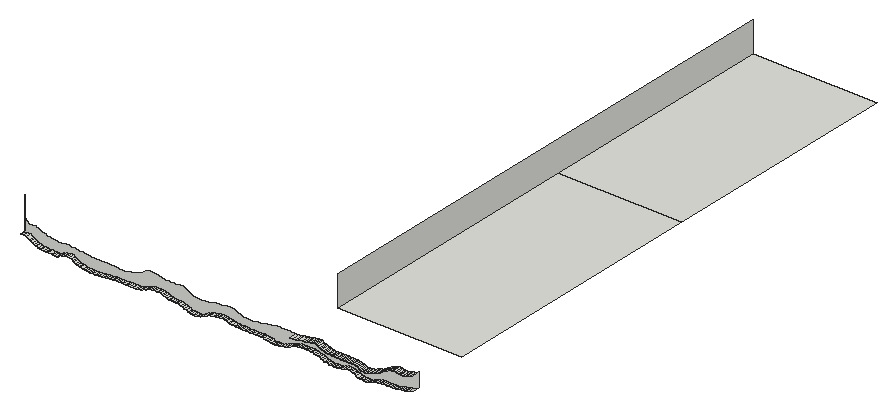
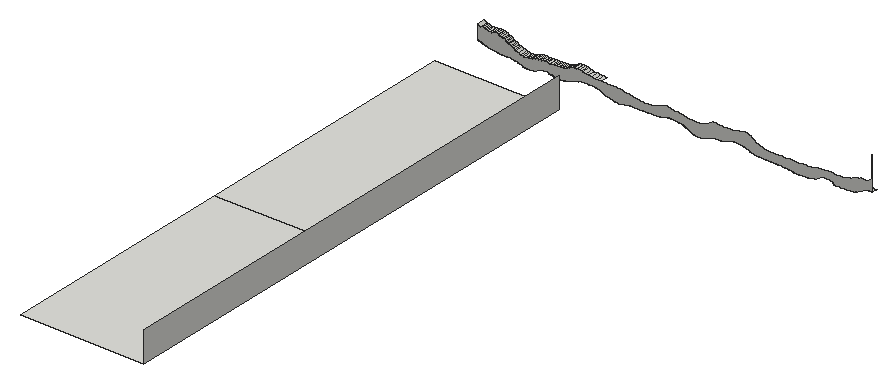
# SketchUp Ruby script. Lengths in inches.
U = 1.inch
M = Sketchup.active_model
def pt(a) = Geom::Point3d.new(a.map { |v| v * U })
def face(e, loops, mat)
  f = e.add_face(loops[0].map { |a| pt(a) })
  loops[1..].each { |l| e.add_face(l.map { |a| pt(a) }).erase! }
  f.material = f.back_material = mat if mat
  f
end
# faces: each face lists its corners as indices into pts; further lists are holes
def faces(e, pts, list, mat = nil) = list.each { |f| face(e, (f[0].is_a?(Array) ? f : [f]).map { |l| l.map { |i| pts[i] } }, mat) }
# xy, xz, yz: faces in a plane at the given z, y or x. An outline is a flat list of corners, or four numbers for a rectangle; further outlines are holes
def ring(l) = l.size == 4 ? [[l[0], l[1]], [l[2], l[1]], [l[2], l[3]], [l[0], l[3]]] : l.each_slice(2).to_a
def flat(e, list, mat, &to3) = list.each { |f| face(e, (f[0].is_a?(Array) ? f : [f]).map { |l| ring(l).map { |u, v| to3.(u, v) } }, mat) }
def xy(e, z, list, mat = nil) = flat(e, list, mat) { |x, y| [x, y, z] }
def xz(e, y, list, mat = nil) = flat(e, list, mat) { |x, z| [x, y, z] }
def yz(e, x, list, mat = nil) = flat(e, list, mat) { |y, z| [x, y, z] }
def lines(e, pts, list) = list.each { |a, b| e.add_line(pt(pts[a]), pt(pts[b])) }
# prism: a flat outline (further loops are holes) pulled along v
def prism(e, loops, v, mat = nil)
  f = face(e, loops, mat); d = Geom::Vector3d.new(v.map { |x| x * U })
  f.pushpull(f.normal.samedirection?(d) ? d.length : -d.length)
end
def box(e, o, s, mat = nil) = prism(e, [[o, [o[0] + s[0], o[1], o[2]], [o[0] + s[0], o[1] + s[1], o[2]], [o[0], o[1] + s[1], o[2]]]], [0, 0, s[2]], mat)
def at(x, y, z, deg = 0) = Geom::Transformation.translation(pt([x, y, z])) * Geom::Transformation.rotation(ORIGIN, Z_AXIS, deg.degrees)
def axes(o, x, y, z) = Geom::Transformation.new([*x, 0, *y, 0, *z, 0, *pt(o).to_a, 1])
def part(name) = M.definitions.add(name)
# library, detail: a bought-in or finely detailed component or shape, given as its bounding box
def library(name, o, s) = part(name).tap { |d| box(d.entities, o, s) }
def detail(e, o, s) = box(e.add_group.entities, o, s)
def put(e, d, t, mat = nil) = e.add_instance(d, t).tap { |i| i.material = mat if mat }
def group(e, t, mat = nil) = e.add_group.tap { |g| g.transformation = t; g.material = mat if mat }.entities
root = M.entities
xy(root,237.65,[[2918.33,2402.3,2919.02,2404.3],[2919.02,2402.3,2919.64,2404.3]])
xy(root,238.18,[[3012.28,2402.3,3012.96,2404.3]])
xy(root,238.33,[[2927.43,2402.3,2927.98,2404.3],[2927.98,2402.3,2928.66,2404.3]])
xy(root,238.34,[[2929.34,2402.3,2930.27,2404.3],[2930.27,2402.3,2930.76,2404.3],[2930.76,2402.3,2931.52,2404.3],[2931.52,2402.3,2932.15,2404.3],[2932.15,2402.3,2932.9,2404.3],
  [2932.9,2402.3,2933.52,2404.3],[2933.52,2402.3,2934.29,2404.3],[2934.29,2402.3,2934.91,2404.3]])
xy(root,238.62,[[2978.81,2402.3,2979.58,2404.3],[2979.58,2402.3,2980.21,2404.3],[2980.21,2402.3,2980.97,2404.3],[2980.97,2402.3,2981.59,2404.3],[2981.59,2402.3,2982.44,2404.3],
  [2982.44,2402.3,2983.08,2404.3],[2983.08,2402.3,2983.7,2404.3]])
xy(root,238.625,[[2977.39,2402.3,2978.25,2404.3]])
xy(root,238.89,[[3033.2,2402.3,3033.88,2404.3]])
xy(root,238.9,[[3034.64,2402.3,3035.26,2404.3],[3035.26,2402.3,3036.03,2404.3]])
xy(root,240.43,[[3001.48,2402.3,3002.05,2404.3]])
xy(root,241.52,[[2889.03,2402.3,2889.09,2404.3]])
xy(root,242.28,[[3019.3,2401.37,3019.8125,2404.3]])
xy(root,242.3,[[3017.54,2401.37,3018.21,2404.3]])
xy(root,242.33,[[3015.13,2401.37,3015.71,2404.3]])
xy(root,242.625,[[2994.64,2425.46,3043.1,2532.83],[2994.64,2532.83,3043.1,2628.15]])
xz(root,2404.3,[[2957.95,236.98,2957.34,237.01,2956.65,237.04,2955.89,237.11,2955.2,237.2,2954.67,237.33,2954,237.68,2953.0625,237.96,2952.5,238.28,2951.72,238.43,2950.94,238.78,2950.27,238.79,2949.73,238.8,2948.97,238.83,2948.22,238.875,2947.65,238.94,2947.07,239.04,2946.41,239.29,2945.83,239.53,2945.3,239.7,2944.61,239.92,2943.98,240.11,2943.2,240.27,2942.58,240.25,2941.875,240.23,2941.11,240.19,2940.4375,240.12,2939.78,240.03,2939.14,239.85,2938.59,239.52,2938.03,239.35,2937.44,239.18,2936.93,238.86,2936.24,238.72,2935.42,238.59,2934.91,238.34,2929.34,238.34,2928.66,238.33,2927.43,238.33,2926.71,238.32,2925.86,238.3,2925.23,238.28,2924.48,238.26,2923.85,238.15,2923.09,238.13,2922.54,238.1,2921.6875,237.98,2921.07,237.94,2920.31,237.89,2919.64,237.65,2918.33,237.65,2917.64,237.66,2916.89,237.67,2916.29,237.68,2915.68,237.71,2914.97,237.76,2914.28,237.82,2913.62,237.9,2912.68,238.21,2912.21,238.31,2911.3,238.43,2910.65,238.74,2910.07,239.11,2909.49,239.38,2909.03,239.71,2908.33,240.11,2907.64,240.09,2906.98,240.05,2906.39,239.99,2905.66,239.88,2905.11,239.69,2904.53,239.55,2903.97,238.9375,2903.44,238.77,2902.7,238.79,2901.83,238.8,2901.32,238.82,2900.28,238.92,2899.59,238.93,2898.89,238.94,2898.19,238.97,2897.51,239.03,2896.82,239.09,2896.04,239.19,2895.53,239.52,2894.97,239.64,2894.52,239.86,2893.73,240.2,2893.13,240.59,2892.59,240.85,2891.57,241.55,2890.3,241.69,2889.09,241.52,2889.09,246.2,2890.66,244.96,2892.05,244.9375,2893.3,244.92,2893.52,244.61,2894.08,244.54,2894.84,244.41,2895.51,244.11,2896.03,243.95,2896.69,243.79,2897.21,243.48,2897.85,243.3,2898.4375,243.14,2898.92,243.06,2899.64,242.85,2900.22,242.78,2901.03,242.73,2901.57,242.68,2902.24,242.51,2902.76,242.46,2903.3,242.58,2903.93,242.57,2904.56,242.81,2905.13,242.86,2905.69,242.89,2906.33,242.92,2906.76,242.625,2907.37,242.65,2907.92,242.62,2908.55,242.58,2909.11,242.57,2909.75,242.48,2910.41,242.38,2911.07,242.34,2911.74,242.24,2912.91,241.96,2913.68,241.89,2914.5,241.83,2915.1,241.78,2915.87,241.75,2916.32,241.74,2916.87,241.72,2918.13,241.7,2918.86,241.69,2919.53,241.68,2920.12,241.68,2920.61,241.67,2921.3125,241.74,2921.88,241.75,2923.88,241.75,2924.37,241.67,2924.9,241.66,2925.51,241.57,2926.05,241.53,2926.67,241.51,2927.22,241.49,2927.92,241.48,2928.58,241.47,2929.15,241.46,2929.86,241.6,2930.59,241.85,2931.26,241.91,2932.16,242.1,2932.93,242.46,2933.63,242.78,2934.4,242.97,2934.93,243.23,2935.33,243.48,2935.85,243.72,2936.1875,244.12,2936.66,244.39,2937.14,244.73,2937.625,244.87,2938.21,244.95,2938.89,245.01,2939.54,244.81,2940.11,244.7,2940.59,244.67,2941.2,244.55,2941.74,244.51,2942.2,244.25,2942.95,244.11,2943.51,244.04,2944.13,243.99,2944.85,243.95,2945.35,243.93,2946.04,243.91,2946.61,243.89,2947.31,243.88,2947.96,243.94,2948.6,243.95,2949.16,244.1,2949.79,244.13,2950.27,244.15,2950.79,244.17,2951.31,244.18,2951.91,243.8,2952.45,243.43,2953.06,243.09,2953.45,242.875,2953.95,242.68,2954.54,242.51,2955.05,242.21,2955.65,242.11,2956.33,241.96,2956.89,241.89,2957.35,241.85,2957.87,241.8125,2958.38,241.79,2958.96,241.78,2959.63,241.91,2960.1,241.93,2960.77,242.09,2961.54,242.2,2962.04,242.24,2962.65,242.42,2963.2,242.47,2963.95,242.71,2964.59,242.78,2965.07,242.82,2965.76,242.85,2966.46,242.87,2967.01,243.02,2967.63,243.05,2968.18,243.29,2968.86,243.35,2969.41,243.39,2970.01,243.42,2970.78,243.14,2971.35,242.9375,2971.9,242.65,2972.52,242.39,2973.28,242.14,2973.92,241.89,2974.41,241.78,2975.46,241.63,2976.23,241.56,2976.83,241.51,2977.28,241.48,2977.8,241.46,2978.67,241.51,2979.39,241.59,2980.33,241.82,2981.11,241.87,2981.875,241.98,2982.49,242.02,2983.14,242.19,2983.84,242.38,2984.33,242.4375,2984.85,242.48,2985.51,242.58,2986.04,242.61,2986.625,242.77,2987.08,242.95,2987.64,243.01,2988.15,243.05,2988.72,243.08,2989.375,243.09,2991.53,243.09,2992.1,243.08,2992.6875,243.07,2993.27,243.07,2993.93,243.0625,2994.54,243.05,2995.22,243.05,2996.49,243.1,2997.66,243.17,2998.8,243.4,3000.0625,243.52,3001.19,243.71,3002.09,243.99,3002.79,244.08,3003.49,244.21,3004.07,244.27,3004.61,244.3,3005.28,244.39,3005.875,244.19,3006.25,243.88,3006.73,243.59,3007.28,243.33,3007.83,243.22,3008.32,242.92,3008.8,242.75,3009.36,242.6,3009.92,242.52,3010.48,242.47,3011.0625,242.43,3011.64,242.4,3012.22,242.39,3012.8,242.37,3013.38,242.36,3013.97,242.35,3015.13,242.33,3015.71,242.33,3016.43,242.32,3016.9,242.3125,3017.54,242.3,3018.21,242.3,3018.66,242.29,3019.3,242.28,3019.8125,242.28,3020.44,242.2,3021.02,241.97,3021.59,241.84,3022.1,241.57,3022.52,241.33,3022.99,241.24,3023.52,241.17,3023.99,241.12,3024.59,241.09,3025.16,241.14,3025.8,241.35,3026.39,241.46,3027.33,241.85,3028.33,242.23,3028.89,242.42,3029.61,242.61,3030.125,242.91,3030.5,243.14,3031.04,243.52,3031.52,243.71,3031.85,244.02,3032.29,244.21,3032.88,244.57,3033.35,244.76,3033.97,245.125,3034.47,245.32,3034.95,245.41,3035.5,245.48,3035.99,245.59,3036.52,245.55,3037.13,245.35,3037.62,245.31,3038.17,245.27,3038.73,245.24,3039.29,245.22,3039.85,245.34,3040.48,245.42,3041.0625,245.52,3041.44,245.76,3041.91,245.9,3043.1,246.43,3043.1,240.89,3041.27,240.1,3040.71,239.96,3040.1875,239.81,3039.5,239.53,3038.95,239.49,3038.23,239.42,3037.43,239.28,3036.66,239.15,3036.03,238.9,3034.64,238.9,3033.88,238.89,3033.2,238.89,3032.52,238.88,3031.98,238.875,3031.22,238.86,3030.48,238.83,3029.91,238.8,3029.33,238.74,3028.67,238.6,3028.1,238.51,3027.57,238.33,3026.88,238.08,3026.2,237.84,3025.51,237.5625,3024.91,237.47,3024.23,237.4,3023.5,237.42,3022.93,237.45,3022.34,237.51,3021.74,237.59,3021.2,237.71,3020.37,238,3019.66,238.33,3019.11,238.57,3018.61,238.86,3018.09,238.96,3017.4,239.02,3016.72,239.125,3015.98,239.04,3015.41,238.66,3014.82,238.61,3014.16,238.55,3013.64,238.27,3012.96,238.18,3012.28,238.18,3011.61,238.11,3011.08,238.15,3010.26,238.19,3009.6875,238.26,3009.12,238.48,3008.46,238.56,3007.89,238.67,3007.37,239.01,3006.6875,239.18,3006.0625,239.5,3005.3,239.65,3004.6875,239.8,3003.93,239.96,3003.28,240.23,3002.7,240.27,3002.05,240.43,3001.48,240.43,3000.9,240.42,3000.375,240.41,2999.68,240.4,2998.99,240.37,2998.3,240.33,2997.62,240.27,2996.94,240.17,2996.32,239.97,2995.67,239.75,2994.93,239.375,2994.14,239.08,2993.26,238.72,2992.51,238.46,2991.29,238.14,2990.17,237.88,2989.52,237.87,2988.65,237.74,2987.94,237.79,2987.17,237.86,2986.54,238.15,2985.77,238.19,2985.15,238.25,2984.39,238.45,2983.7,238.62,2978.81,238.62,2978.25,238.625,2977.39,238.625,2976.7,238.63,2976.08,238.64,2975.3,238.65,2974.63,238.66,2973.94,238.6875,2973.27,238.73,2972.79,238.78,2971.91,238.93,2971.14,239.07,2970.59,239.16,2969.74,239.44,2969.07,239.56,2968.46,239.72,2967.73,239.7,2967.17,239.69,2966.58,239.65,2965.96,239.6,2965.47,239.54,2964.66,239.31,2963.66,239.22,2963.08,239.12,2962.4375,238.76,2961.8,238.51,2961.24,238.375,2960.8,238.02,2960.1,237.74,2959.48,237.43,2958.63,237.22],[2889.03,241.52,2889.09,254.5]])
yz(root,2994.64,[[2425.46,242.625,2628.15,254.5]])
p = [[2955.89,2404.3,237.11],[2956.65,2404.3,237.04],[2956.65,2402.3,237.04],[2955.89,2402.3,237.11],[2957.34,2404.3,237.01],[2957.34,2402.3,237.01],
  [2957.95,2404.3,236.98],[2957.95,2402.3,236.98],[2958.63,2404.3,237.22],[2958.63,2402.3,237.22],[2955.2,2404.3,237.2],[2955.2,2402.3,237.2],
  [2954.67,2404.3,237.33],[2954.67,2402.3,237.33],[2959.48,2404.3,237.43],[2959.48,2402.3,237.43],[2954,2404.3,237.68],[2954,2402.3,237.68],
  [2960.1,2404.3,237.74],[2960.1,2402.3,237.74],[3022.93,2404.3,237.45],[3023.5,2404.3,237.42],[3023.5,2402.3,237.42],[3022.93,2402.3,237.45],
  [3024.23,2404.3,237.4],[3024.23,2402.3,237.4],[3024.91,2404.3,237.47],[3024.91,2402.3,237.47],[3021.74,2404.3,237.59],[3022.34,2404.3,237.51],
  [3022.34,2402.3,237.51],[3021.74,2402.3,237.59],[3025.51,2404.3,237.5625],[3025.51,2402.3,237.5625],[2919.64,2404.3,237.65],[2920.31,2404.3,237.89],
  [2920.31,2402.3,237.89],[2919.64,2402.3,237.65],[3021.2,2404.3,237.71],[3021.2,2402.3,237.71],[3026.2,2404.3,237.84],[3026.2,2402.3,237.84],
  [2914.97,2404.3,237.76],[2915.68,2404.3,237.71],[2915.68,2402.3,237.71],[2914.97,2402.3,237.76],[2916.29,2404.3,237.68],[2916.29,2402.3,237.68],
  [2916.89,2404.3,237.67],[2916.89,2402.3,237.67],[2917.64,2404.3,237.66],[2917.64,2402.3,237.66],[2918.33,2404.3,237.65],[2918.33,2402.3,237.65],
  [2953.0625,2404.3,237.96],[2953.0625,2402.3,237.96],[2960.8,2404.3,238.02],[2960.8,2402.3,238.02],[2987.94,2404.3,237.79],[2988.65,2404.3,237.74],
  [2988.65,2402.3,237.74],[2987.94,2402.3,237.79],[2989.52,2404.3,237.87],[2989.52,2402.3,237.87],[3020.37,2404.3,238],[3020.37,2402.3,238],
  [2913.62,2404.3,237.9],[2914.28,2404.3,237.82],[2914.28,2402.3,237.82],[2913.62,2402.3,237.9],[2987.17,2404.3,237.86],[2987.17,2402.3,237.86],
  [3026.88,2404.3,238.08],[3026.88,2402.3,238.08],[2912.68,2404.3,238.21],[2912.68,2402.3,238.21],[2921.07,2404.3,237.94],[2921.07,2402.3,237.94],
  [2921.6875,2404.3,237.98],[2921.6875,2402.3,237.98],[2986.54,2404.3,238.15],[2986.54,2402.3,238.15],[2990.17,2404.3,237.88],[2990.17,2402.3,237.88],
  [2991.29,2404.3,238.14],[2991.29,2402.3,238.14],[2922.54,2404.3,238.1],[2922.54,2402.3,238.1],[2952.5,2404.3,238.28],[2952.5,2402.3,238.28],
  [2961.24,2404.3,238.375],[2961.24,2402.3,238.375],[3019.66,2404.3,238.33],[3019.66,2402.3,238.33],[2923.09,2404.3,238.13],[2923.09,2402.3,238.13],
  [2923.85,2404.3,238.15],[2923.85,2402.3,238.15],[2985.77,2404.3,238.19],[2985.77,2402.3,238.19],[2992.51,2404.3,238.46],[2992.51,2402.3,238.46],
  [3010.26,2404.3,238.19],[3011.08,2404.3,238.15],[3011.08,2402.3,238.15],[3010.26,2402.3,238.19],[3011.61,2404.3,238.11],[3011.61,2402.3,238.11],
  [3012.28,2404.3,238.18],[3012.28,2402.3,238.18],[3027.57,2404.3,238.33],[3027.57,2402.3,238.33],[2912.21,2404.3,238.31],[2912.21,2402.3,238.31],
  [2924.48,2404.3,238.26],[2924.48,2402.3,238.26],[2985.15,2404.3,238.25],[2985.15,2402.3,238.25],[3009.6875,2404.3,238.26],[3009.6875,2402.3,238.26],
  [3012.96,2404.3,238.18],[3013.64,2404.3,238.27],[3013.64,2402.3,238.27],[3012.96,2402.3,238.18],[2911.3,2404.3,238.43],[2911.3,2402.3,238.43],
  [2925.23,2404.3,238.28],[2925.23,2402.3,238.28],[2925.86,2404.3,238.3],[2925.86,2402.3,238.3],[2926.71,2404.3,238.32],[2926.71,2402.3,238.32],
  [2927.43,2404.3,238.33],[2927.43,2402.3,238.33],[2928.66,2404.3,238.33],[2929.34,2404.3,238.34],[2929.34,2402.3,238.34],[2928.66,2402.3,238.33],
  [2934.91,2404.3,238.34],[2935.42,2404.3,238.59],[2935.42,2402.3,238.59],[2934.91,2402.3,238.34],[2951.72,2404.3,238.43],[2951.72,2402.3,238.43],
  [2984.39,2404.3,238.45],[2984.39,2402.3,238.45],[3009.12,2404.3,238.48],[3009.12,2402.3,238.48],[3014.16,2404.3,238.55],[3014.16,2402.3,238.55],
  [3019.11,2404.3,238.57],[3019.11,2402.3,238.57],[3028.1,2404.3,238.51],[3028.1,2402.3,238.51],[2910.65,2404.3,238.74],[2910.65,2402.3,238.74],
  [2950.94,2404.3,238.78],[2950.94,2402.3,238.78],[2961.8,2404.3,238.51],[2961.8,2402.3,238.51],[2962.4375,2404.3,238.76],[2962.4375,2402.3,238.76],
  [2983.7,2404.3,238.62],[2983.7,2402.3,238.62],[2993.26,2404.3,238.72],[2993.26,2402.3,238.72],[3008.46,2404.3,238.56],[3008.46,2402.3,238.56],
  [3014.82,2404.3,238.61],[3014.82,2402.3,238.61],[3028.67,2404.3,238.6],[3028.67,2402.3,238.6],[2936.24,2404.3,238.72],[2936.24,2402.3,238.72],
  [2974.63,2404.3,238.66],[2975.3,2404.3,238.65],[2975.3,2402.3,238.65],[2974.63,2402.3,238.66],[2976.08,2404.3,238.64],[2976.08,2402.3,238.64],
  [2976.7,2404.3,238.63],[2976.7,2402.3,238.63],[2977.39,2404.3,238.625],[2977.39,2402.3,238.625],[2978.25,2404.3,238.625],[2978.81,2404.3,238.62],
  [2978.81,2402.3,238.62],[2978.25,2402.3,238.625],[3007.89,2404.3,238.67],[3007.89,2402.3,238.67],[3015.41,2404.3,238.66],[3015.41,2402.3,238.66],
  [3018.61,2404.3,238.86],[3018.61,2402.3,238.86],[3029.33,2404.3,238.74],[3029.33,2402.3,238.74],[2910.07,2404.3,239.11],[2910.07,2402.3,239.11],
  [2936.93,2404.3,238.86],[2936.93,2402.3,238.86],[2972.79,2404.3,238.78],[2973.27,2404.3,238.73],[2973.27,2402.3,238.73],[2972.79,2402.3,238.78],
  [2973.94,2404.3,238.6875],[2973.94,2402.3,238.6875],[2994.14,2404.3,239.08],[2994.14,2402.3,239.08],[3007.37,2404.3,239.01],[3007.37,2402.3,239.01],
  [3015.98,2404.3,239.04],[3015.98,2402.3,239.04],[3029.91,2404.3,238.8],[3029.91,2402.3,238.8],[2900.28,2404.3,238.92],[2901.32,2404.3,238.82],
  [2901.32,2402.3,238.82],[2900.28,2402.3,238.92],[2901.83,2404.3,238.8],[2901.83,2402.3,238.8],[2902.7,2404.3,238.79],[2902.7,2402.3,238.79],
  [2903.44,2404.3,238.77],[2903.44,2402.3,238.77],[2903.97,2404.3,238.9375],[2903.97,2402.3,238.9375],[2948.22,2404.3,238.875],[2948.97,2404.3,238.83],
  [2948.97,2402.3,238.83],[2948.22,2402.3,238.875],[2949.73,2404.3,238.8],[2949.73,2402.3,238.8],[2950.27,2404.3,238.79],[2950.27,2402.3,238.79],
  [2963.08,2404.3,239.12],[2963.08,2402.3,239.12],[2971.91,2404.3,238.93],[2971.91,2402.3,238.93],[3030.48,2404.3,238.83],[3030.48,2402.3,238.83],
  [3031.22,2404.3,238.86],[3031.22,2402.3,238.86],[2898.19,2404.3,238.97],[2898.89,2404.3,238.94],[2898.89,2402.3,238.94],[2898.19,2402.3,238.97],
  [2899.59,2404.3,238.93],[2899.59,2402.3,238.93],[2904.53,2404.3,239.55],[2904.53,2402.3,239.55],[2937.44,2404.3,239.18],[2937.44,2402.3,239.18],
  [2947.07,2404.3,239.04],[2947.65,2404.3,238.94],[2947.65,2402.3,238.94],[2947.07,2402.3,239.04],[2971.14,2404.3,239.07],[2971.14,2402.3,239.07],
  [3018.09,2404.3,238.96],[3018.09,2402.3,238.96],[3031.98,2404.3,238.875],[3031.98,2402.3,238.875],[3032.52,2404.3,238.88],[3032.52,2402.3,238.88],
  [3033.2,2404.3,238.89],[3033.2,2402.3,238.89],[3033.88,2404.3,238.89],[3034.64,2404.3,238.9],[3034.64,2402.3,238.9],[3033.88,2402.3,238.89],
  [3036.03,2404.3,238.9],[3036.66,2404.3,239.15],[3036.66,2402.3,239.15],[3036.03,2402.3,238.9],[2896.82,2404.3,239.09],[2897.51,2404.3,239.03],
  [2897.51,2402.3,239.03],[2896.82,2402.3,239.09],[2946.41,2404.3,239.29],[2946.41,2402.3,239.29],[3006.6875,2404.3,239.18],[3006.6875,2402.3,239.18],
  [3016.72,2404.3,239.125],[3016.72,2402.3,239.125],[3017.4,2404.3,239.02],[3017.4,2402.3,239.02],[2896.04,2404.3,239.19],[2896.04,2402.3,239.19],
  [2909.49,2404.3,239.38],[2909.49,2402.3,239.38],[2963.66,2404.3,239.22],[2963.66,2402.3,239.22],[2970.59,2404.3,239.16],[2970.59,2402.3,239.16],
  [2994.93,2404.3,239.375],[2994.93,2402.3,239.375],[2895.53,2404.3,239.52],[2895.53,2402.3,239.52],[2938.03,2404.3,239.35],[2938.03,2402.3,239.35],
  [2964.66,2404.3,239.31],[2964.66,2402.3,239.31],[2969.74,2404.3,239.44],[2969.74,2402.3,239.44],[3006.0625,2404.3,239.5],[3006.0625,2402.3,239.5],
  [3037.43,2404.3,239.28],[3037.43,2402.3,239.28],[2945.83,2404.3,239.53],[2945.83,2402.3,239.53],[2965.47,2404.3,239.54],[2965.47,2402.3,239.54],
  [3038.23,2404.3,239.42],[3038.23,2402.3,239.42],[2909.03,2404.3,239.71],[2909.03,2402.3,239.71],[2938.59,2404.3,239.52],[2938.59,2402.3,239.52],
  [2969.07,2404.3,239.56],[2969.07,2402.3,239.56],[2995.67,2404.3,239.75],[2995.67,2402.3,239.75],[3038.95,2404.3,239.49],[3038.95,2402.3,239.49],
  [2894.97,2404.3,239.64],[2894.97,2402.3,239.64],[2939.14,2404.3,239.85],[2939.14,2402.3,239.85],[2945.3,2404.3,239.7],[2945.3,2402.3,239.7],
  [2965.96,2404.3,239.6],[2965.96,2402.3,239.6],[3005.3,2404.3,239.65],[3005.3,2402.3,239.65],[3039.5,2404.3,239.53],[3039.5,2402.3,239.53],
  [3040.1875,2404.3,239.81],[3040.1875,2402.3,239.81],[2894.52,2404.3,239.86],[2894.52,2402.3,239.86],[2905.11,2404.3,239.69],[2905.11,2402.3,239.69],
  [2966.58,2404.3,239.65],[2966.58,2402.3,239.65],[2967.17,2404.3,239.69],[2967.17,2402.3,239.69],[2968.46,2404.3,239.72],[2968.46,2402.3,239.72],
  [2905.66,2404.3,239.88],[2905.66,2402.3,239.88],[2908.33,2404.3,240.11],[2908.33,2402.3,240.11],[2944.61,2404.3,239.92],[2944.61,2402.3,239.92],
  [2967.73,2404.3,239.7],[2967.73,2402.3,239.7],[2996.32,2404.3,239.97],[2996.32,2402.3,239.97],[3004.6875,2404.3,239.8],[3004.6875,2402.3,239.8],
  [2939.78,2404.3,240.03],[2939.78,2402.3,240.03],[3003.93,2404.3,239.96],[3003.93,2402.3,239.96],[3040.71,2404.3,239.96],[3040.71,2402.3,239.96],
  [2893.73,2404.3,240.2],[2893.73,2402.3,240.2],[2906.39,2404.3,239.99],[2906.39,2402.3,239.99],[2943.98,2404.3,240.11],[2943.98,2402.3,240.11],
  [2906.98,2404.3,240.05],[2906.98,2402.3,240.05],[2907.64,2404.3,240.09],[2907.64,2402.3,240.09],[2940.4375,2404.3,240.12],[2940.4375,2402.3,240.12],
  [2996.94,2404.3,240.17],[2996.94,2402.3,240.17],[3003.28,2404.3,240.23],[3003.28,2402.3,240.23],[3041.27,2404.3,240.1],[3041.27,2402.3,240.1],
  [2941.11,2404.3,240.19],[2941.11,2402.3,240.19],[2943.2,2404.3,240.27],[2943.2,2402.3,240.27],[3043.1,2404.3,240.89],[3043.1,2402.3,240.89],
  [2893.13,2404.3,240.59],[2893.13,2402.3,240.59],[2941.875,2404.3,240.23],[2941.875,2402.3,240.23],[2942.58,2404.3,240.25],[2942.58,2402.3,240.25],
  [2997.62,2404.3,240.27],[2997.62,2402.3,240.27],[3002.7,2404.3,240.27],[3002.7,2402.3,240.27],[2998.3,2404.3,240.33],[2998.3,2402.3,240.33],
  [2998.99,2404.3,240.37],[2998.99,2402.3,240.37],[3002.05,2404.3,240.43],[3002.05,2402.3,240.43],[2999.68,2404.3,240.4],[2999.68,2402.3,240.4],
  [3000.375,2404.3,240.41],[3000.375,2402.3,240.41],[3000.9,2404.3,240.42],[3000.9,2402.3,240.42],[3001.48,2404.3,240.43],[3001.48,2402.3,240.43],
  [2892.59,2404.3,240.85],[2892.59,2402.3,240.85],[2891.57,2404.3,241.55],[2891.57,2402.3,241.55],[3023.52,2404.3,241.17],[3023.99,2404.3,241.12],
  [3023.99,2401.37,241.12],[3023.52,2401.37,241.17],[3024.59,2404.3,241.09],[3024.59,2401.37,241.09],[3025.16,2404.3,241.14],[3025.16,2401.37,241.14],
  [3025.8,2404.3,241.35],[3025.8,2401.37,241.35],[3022.52,2404.3,241.33],[3022.99,2404.3,241.24],[3022.99,2401.37,241.24],[3022.52,2401.37,241.33],
  [3022.1,2404.3,241.57],[3022.1,2401.37,241.57],[3026.39,2404.3,241.46],[3026.39,2401.37,241.46],[3027.33,2404.3,241.85],[3027.33,2401.37,241.85],
  [2889.09,2404.3,241.52],[2890.3,2404.3,241.69],[2890.3,2402.3,241.69],[2889.09,2402.3,241.52],[3021.59,2404.3,241.84],[3021.59,2401.37,241.84],
  [3021.02,2404.3,241.97],[3021.02,2401.37,241.97],[3028.33,2404.3,242.23],[3028.33,2401.37,242.23],[3020.44,2404.3,242.2],[3020.44,2401.37,242.2],
  [3019.8125,2404.3,242.28],[3019.8125,2401.37,242.28],[3028.89,2404.3,242.42],[3028.89,2401.37,242.42],[3013.97,2404.3,242.35],[3014.55,2404.3,242.34],
  [3014.55,2401.37,242.34],[3013.97,2401.37,242.35],[3015.13,2404.3,242.33],[3015.13,2401.37,242.33],[3015.71,2404.3,242.33],[3016.43,2404.3,242.32],
  [3016.43,2401.37,242.32],[3015.71,2401.37,242.33],[3016.9,2404.3,242.3125],[3016.9,2401.37,242.3125],[3017.54,2404.3,242.3],[3017.54,2401.37,242.3],
  [3018.21,2404.3,242.3],[3018.66,2404.3,242.29],[3018.66,2401.37,242.29],[3018.21,2401.37,242.3],[3019.3,2404.3,242.28],[3019.3,2401.37,242.28],
  [3010.48,2404.3,242.47],[3011.0625,2404.3,242.43],[3011.0625,2401.37,242.43],[3010.48,2401.37,242.47],[3011.64,2404.3,242.4],[3011.64,2401.37,242.4],
  [3012.22,2404.3,242.39],[3012.22,2401.37,242.39],[3012.8,2404.3,242.37],[3012.8,2401.37,242.37],[3013.38,2404.3,242.36],[3013.38,2401.37,242.36],
  [3029.61,2404.3,242.61],[3029.61,2401.37,242.61],[3009.36,2404.3,242.6],[3009.92,2404.3,242.52],[3009.92,2401.37,242.52],[3009.36,2401.37,242.6],
  [3008.8,2404.3,242.75],[3008.8,2401.37,242.75],[3030.125,2404.3,242.91],[3030.125,2401.37,242.91],[3008.32,2404.3,242.92],[3008.32,2401.37,242.92],
  [3007.83,2404.3,243.22],[3007.83,2401.37,243.22],[3030.5,2404.3,243.14],[3030.5,2401.37,243.14],[2995.22,2404.3,243.05],[2996.49,2404.3,243.1],
  [2996.49,2401.37,243.1],[2995.22,2401.37,243.05],[2997.66,2404.3,243.17],[2997.66,2401.37,243.17],[3031.04,2404.3,243.52],[3031.04,2401.37,243.52],
  [2998.8,2404.3,243.4],[2998.8,2401.37,243.4],[3007.28,2404.3,243.33],[3007.28,2401.37,243.33],[3006.73,2404.3,243.59],[3006.73,2401.37,243.59],
  [3000.0625,2404.3,243.52],[3000.0625,2401.37,243.52],[3001.19,2404.3,243.71],[3001.19,2401.37,243.71],[3031.52,2404.3,243.71],[3031.52,2401.37,243.71],
  [3006.25,2404.3,243.88],[3006.25,2401.37,243.88],[3002.09,2404.3,243.99],[3002.09,2401.37,243.99],[3031.85,2404.3,244.02],[3031.85,2401.37,244.02],
  [3005.875,2404.3,244.19],[3005.875,2401.37,244.19],[3002.79,2404.3,244.08],[3002.79,2401.37,244.08],[3032.29,2404.3,244.21],[3032.29,2401.37,244.21],
  [3003.49,2404.3,244.21],[3003.49,2401.37,244.21],[3004.07,2404.3,244.27],[3004.07,2401.37,244.27],[3005.28,2404.3,244.39],[3005.28,2401.37,244.39],
  [3032.88,2404.3,244.57],[3032.88,2401.37,244.57],[3004.61,2404.3,244.3],[3004.61,2401.37,244.3],[3033.35,2404.3,244.76],[3033.35,2401.37,244.76],
  [3033.97,2404.3,245.125],[3033.97,2401.37,245.125],[3034.47,2404.3,245.32],[3034.47,2401.37,245.32],[3038.17,2404.3,245.27],[3038.73,2404.3,245.24],
  [3038.73,2401.37,245.24],[3038.17,2401.37,245.27],[3039.29,2404.3,245.22],[3039.29,2401.37,245.22],[3039.85,2404.3,245.34],[3039.85,2401.37,245.34],
  [3034.95,2404.3,245.41],[3034.95,2401.37,245.41],[3036.52,2404.3,245.55],[3037.13,2404.3,245.35],[3037.13,2401.37,245.35],[3036.52,2401.37,245.55],
  [3037.62,2404.3,245.31],[3037.62,2401.37,245.31],[3040.48,2404.3,245.42],[3040.48,2401.37,245.42],[3035.5,2404.3,245.48],[3035.5,2401.37,245.48],
  [3041.0625,2404.3,245.52],[3041.0625,2401.37,245.52],[3035.99,2404.3,245.59],[3035.99,2401.37,245.59],[3041.44,2404.3,245.76],[3041.44,2401.37,245.76],
  [3041.91,2404.3,245.9],[3041.91,2401.37,245.9],[3043.1,2404.3,246.43],[3043.1,2401.37,246.43]]
faces(root,p,[[0,1,2,3],[1,4,5,2],[4,6,7,5],[6,8,9,7],[10,0,3,11],[12,10,11,13],[8,14,15,9],[16,12,13,17],
  [14,18,19,15],[20,21,22,23],[21,24,25,22],[24,26,27,25],[28,29,30,31],[29,20,23,30],[26,32,33,27],[34,35,36,37],
  [38,28,31,39],[32,40,41,33],[42,43,44,45],[43,46,47,44],[46,48,49,47],[48,50,51,49],[50,52,53,51],[54,16,17,55],
  [18,56,57,19],[58,59,60,61],[59,62,63,60],[64,38,39,65],[66,67,68,69],[67,42,45,68],[70,58,61,71],[40,72,73,41],
  [74,66,69,75],[35,76,77,36],[76,78,79,77],[80,70,71,81],[62,82,83,63],[82,84,85,83],[78,86,87,79],[88,54,55,89],
  [56,90,91,57],[92,64,65,93],[86,94,95,87],[94,96,97,95],[98,80,81,99],[84,100,101,85],[102,103,104,105],[103,106,107,104],
  [106,108,109,107],[72,110,111,73],[112,74,75,113],[96,114,115,97],[116,98,99,117],[118,102,105,119],[120,121,122,123],[124,112,113,125],
  [114,126,127,115],[126,128,129,127],[128,130,131,129],[130,132,133,131],[134,135,136,137],[138,139,140,141],[142,88,89,143],[144,116,117,145],
  [146,118,119,147],[121,148,149,122],[150,92,93,151],[110,152,153,111],[154,124,125,155],[156,142,143,157],[90,158,159,91],[158,160,161,159],
  [162,144,145,163],[100,164,165,101],[166,146,147,167],[148,168,169,149],[152,170,171,153],[139,172,173,140],[174,175,176,177],[175,178,179,176],
  [178,180,181,179],[180,182,183,181],[184,185,186,187],[188,166,167,189],[168,190,191,169],[192,150,151,193],[170,194,195,171],[196,154,155,197],
  [172,198,199,173],[200,201,202,203],[201,204,205,202],[204,174,177,205],[164,206,207,165],[208,188,189,209],[190,210,211,191],[194,212,213,195],
  [214,215,216,217],[215,218,219,216],[218,220,221,219],[220,222,223,221],[222,224,225,223],[226,227,228,229],[227,230,231,228],[230,232,233,231],
  [232,156,157,233],[160,234,235,161],[236,200,203,237],[212,238,239,213],[238,240,241,239],[242,243,244,245],[243,246,247,244],[246,214,217,247],
  [224,248,249,225],[198,250,251,199],[252,253,254,255],[253,226,229,254],[256,236,237,257],[258,192,193,259],[240,260,261,241],[260,262,263,261],
  [262,264,265,263],[266,267,268,269],[270,271,272,273],[274,275,276,277],[275,242,245,276],[278,252,255,279],[280,208,209,281],[210,282,283,211],
  [282,284,285,283],[284,258,259,285],[286,274,277,287],[288,196,197,289],[234,290,291,235],[292,256,257,293],[206,294,295,207],[296,286,287,297],
  [250,298,299,251],[290,300,301,291],[302,292,293,303],[304,280,281,305],[271,306,307,272],[308,278,279,309],[300,310,311,301],[306,312,313,307],
  [314,288,289,315],[298,316,317,299],[318,302,303,319],[294,320,321,295],[312,322,323,313],[324,296,297,325],[316,326,327,317],[328,308,309,329],
  [310,330,331,311],[332,304,305,333],[322,334,335,323],[334,336,337,335],[338,324,325,339],[248,340,341,249],[330,342,343,331],[342,344,345,343],
  [346,318,319,347],[340,348,349,341],[350,314,315,351],[352,328,329,353],[344,354,355,345],[354,346,347,355],[320,356,357,321],[358,332,333,359],
  [326,360,361,327],[362,358,359,363],[336,364,365,337],[366,338,339,367],[348,368,369,349],[370,352,353,371],[368,372,373,369],[372,374,375,373],
  [360,376,377,361],[356,378,379,357],[380,362,363,381],[364,382,383,365],[374,350,351,375],[376,384,385,377],[386,370,371,387],[382,388,389,383],
  [390,366,367,391],[384,392,393,385],[392,394,395,393],[378,396,397,379],[398,380,381,399],[394,386,387,395],[396,400,401,397],[400,402,403,401],
  [404,398,399,405],[402,406,407,403],[406,408,409,407],[408,410,411,409],[410,412,413,411],[414,390,391,415],[416,414,415,417],[418,419,420,421],
  [419,422,423,420],[422,424,425,423],[424,426,427,425],[428,429,430,431],[429,418,421,430],[432,428,431,433],[426,434,435,427],[434,436,437,435],
  [438,439,440,441],[442,432,433,443],[439,416,417,440],[444,442,443,445],[436,446,447,437],[448,444,445,449],[450,448,449,451],[446,452,453,447],
  [454,455,456,457],[455,458,459,456],[460,461,462,463],[461,464,465,462],[464,466,467,465],[468,469,470,471],[469,472,473,470],[474,475,476,477],
  [475,478,479,476],[478,480,481,479],[480,482,483,481],[482,484,485,483],[484,454,457,485],[452,486,487,453],[488,489,490,491],[489,474,477,490],
  [492,488,491,493],[486,494,495,487],[496,492,493,497],[498,496,497,499],[494,500,501,495],[502,503,504,505],[503,506,507,504],[500,508,509,501],
  [506,510,511,507],[512,498,499,513],[514,512,513,515],[510,516,517,511],[516,518,519,517],[508,520,521,509],[522,514,515,523],[518,524,525,519],
  [520,526,527,521],[528,522,523,529],[524,530,531,525],[526,532,533,527],[530,534,535,531],[534,536,537,535],[538,528,529,539],[532,540,541,533],
  [536,542,543,537],[542,538,539,543],[540,544,545,541],[544,546,547,545],[546,548,549,547],[550,551,552,553],[551,554,555,552],[554,556,557,555],
  [548,558,559,549],[560,561,562,563],[561,564,565,562],[564,550,553,565],[556,566,567,557],[558,568,569,559],[566,570,571,567],[568,572,573,569],
  [570,574,575,571],[572,560,563,573],[574,576,577,575],[576,578,579,577]])
